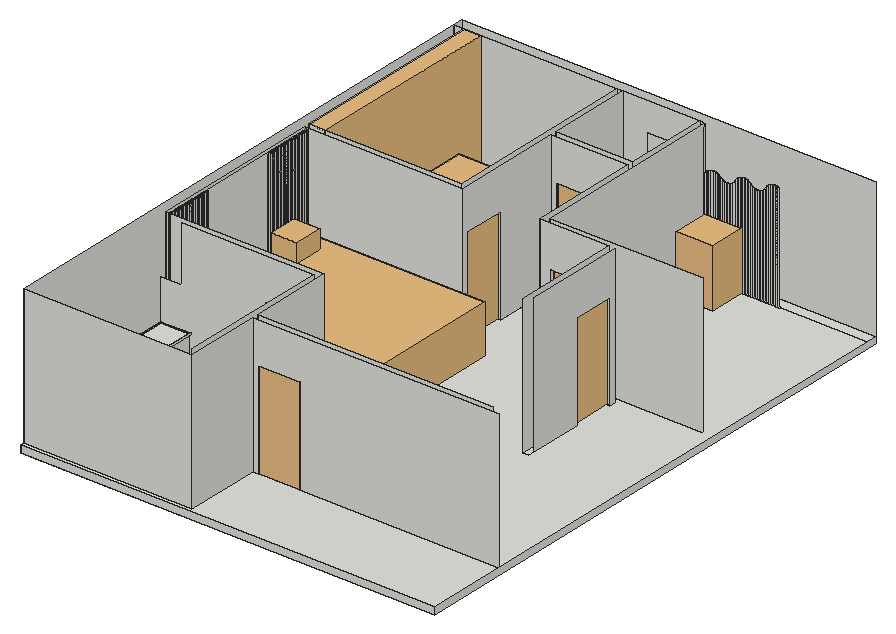
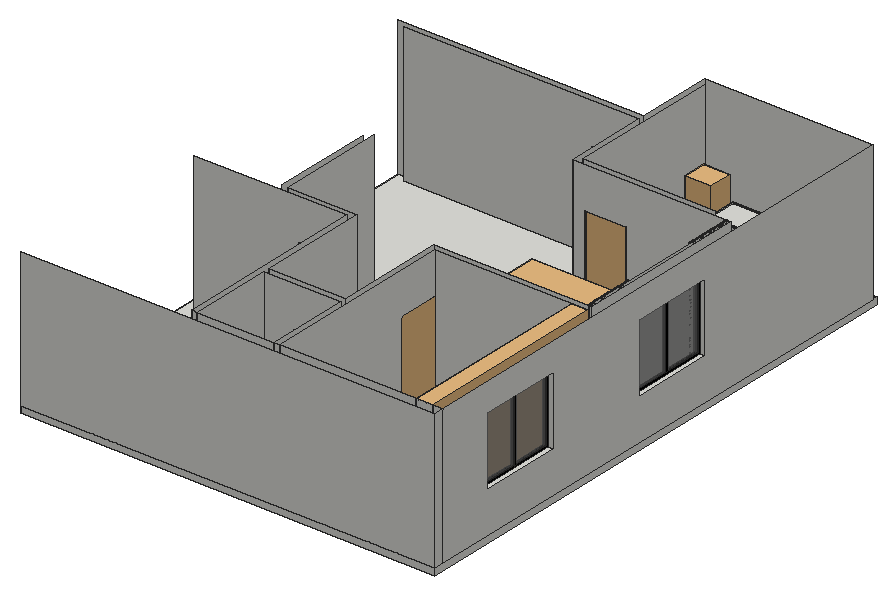
# SketchUp Ruby script. Lengths in inches.
U = 1.inch
M = Sketchup.active_model
def pt(a) = Geom::Point3d.new(a.map { |v| v * U })
def face(e, loops, mat)
  f = e.add_face(loops[0].map { |a| pt(a) })
  loops[1..].each { |l| e.add_face(l.map { |a| pt(a) }).erase! }
  f.material = f.back_material = mat if mat
  f
end
# faces: each face lists its corners as indices into pts; further lists are holes
def faces(e, pts, list, mat = nil) = list.each { |f| face(e, (f[0].is_a?(Array) ? f : [f]).map { |l| l.map { |i| pts[i] } }, mat) }
# xy, xz, yz: faces in a plane at the given z, y or x. An outline is a flat list of corners, or four numbers for a rectangle; further outlines are holes
def ring(l) = l.size == 4 ? [[l[0], l[1]], [l[2], l[1]], [l[2], l[3]], [l[0], l[3]]] : l.each_slice(2).to_a
def flat(e, list, mat, &to3) = list.each { |f| face(e, (f[0].is_a?(Array) ? f : [f]).map { |l| ring(l).map { |u, v| to3.(u, v) } }, mat) }
def xy(e, z, list, mat = nil) = flat(e, list, mat) { |x, y| [x, y, z] }
def xz(e, y, list, mat = nil) = flat(e, list, mat) { |x, z| [x, y, z] }
def yz(e, x, list, mat = nil) = flat(e, list, mat) { |y, z| [x, y, z] }
def lines(e, pts, list) = list.each { |a, b| e.add_line(pt(pts[a]), pt(pts[b])) }
# prism: a flat outline (further loops are holes) pulled along v
def prism(e, loops, v, mat = nil)
  f = face(e, loops, mat); d = Geom::Vector3d.new(v.map { |x| x * U })
  f.pushpull(f.normal.samedirection?(d) ? d.length : -d.length)
end
def box(e, o, s, mat = nil) = prism(e, [[o, [o[0] + s[0], o[1], o[2]], [o[0] + s[0], o[1] + s[1], o[2]], [o[0], o[1] + s[1], o[2]]]], [0, 0, s[2]], mat)
def at(x, y, z, deg = 0) = Geom::Transformation.translation(pt([x, y, z])) * Geom::Transformation.rotation(ORIGIN, Z_AXIS, deg.degrees)
def axes(o, x, y, z) = Geom::Transformation.new([*x, 0, *y, 0, *z, 0, *pt(o).to_a, 1])
def part(name) = M.definitions.add(name)
# library, detail: a bought-in or finely detailed component or shape, given as its bounding box
def library(name, o, s) = part(name).tap { |d| box(d.entities, o, s) }
def detail(e, o, s) = box(e.add_group.entities, o, s)
def put(e, d, t, mat = nil) = e.add_instance(d, t).tap { |i| i.material = mat if mat }
def group(e, t, mat = nil) = e.add_group.tap { |g| g.transformation = t; g.material = mat if mat }.entities
root = M.entities
M.materials.add("[Color_008]").color = [30, 30, 30]
M.materials.add("[Color_009]").color = [0, 0, 0]
M.materials.add("[Translucent_Glass_Gray]").color = [128, 128, 128]
M.materials["[Translucent_Glass_Gray]"].alpha = 0.5
c1 = part("Group\#1")
xy(c1.entities,0,[[0,0,82.68,1.18]],"[Color_009]")
xy(c1.entities,1.97,[[1.97,0.98,40.35,1.18],[42.32,0.98,80.71,1.18]])
xy(c1.entities,1.97,[[1.97,0,40.35,0.3],[42.32,0,80.71,0.3]],"[Color_009]")
xy(c1.entities,80.71,[[1.97,0,40.35,0.3],[42.32,0,80.71,0.3],[1.97,0.3,40.35,0.98],[42.32,0.3,80.71,0.98],[1.97,0.98,40.35,1.18],
  [42.32,0.98,80.71,1.18]])
xy(c1.entities,82.68,[[0,0,82.68,1.18]],"[Color_008]")
xz(c1.entities,0,[[[0,0,82.68,82.68],[1.97,1.97,40.35,80.71],[42.32,1.97,80.71,80.71]]],"[Color_009]")
xz(c1.entities,0.3,[[1.97,1.97,40.35,80.71],[42.32,1.97,80.71,80.71]],"[Translucent_Glass_Gray]")
xz(c1.entities,0.98,[[1.97,1.97,40.35,80.71],[42.32,1.97,80.71,80.71]],"[Translucent_Glass_Gray]")
xz(c1.entities,1.18,[[[0,0,82.68,82.68],[1.97,1.97,80.71,80.71]],[40.35,1.97,42.32,80.71]],"[Color_009]")
yz(c1.entities,0,[[0,0,1.18,82.68]],"[Color_009]")
yz(c1.entities,1.97,[[0.98,1.97,1.18,80.71]])
yz(c1.entities,1.97,[[0,1.97,0.3,80.71]],"[Color_009]")
yz(c1.entities,40.35,[[0,1.97,0.3,80.71],[0.98,1.97,1.18,80.71]],"[Color_009]")
yz(c1.entities,42.32,[[0,1.97,0.3,80.71],[0.98,1.97,1.18,80.71]])
yz(c1.entities,80.71,[[0,1.97,0.3,80.71],[0.98,1.97,1.18,80.71]],"[Color_009]")
yz(c1.entities,82.68,[[0,0,1.18,82.68]],"[Color_009]")
c2 = library("Curtain set",[2.63,-1.5,0.02],[153.32,14.06,114.15])
c3 = part("Vertical slat \#1")
box(c3.entities,[0,0,-18],[1,1,114])
c4 = part("Vertical slat")
box(c4.entities,[0,0,0],[1,1,96])
c5 = library("SKT_Nearly Natural 5' Kentia Palm Silk Tree",[-23.18,-17.61,0],[47.48,43.95,59.125])
c6 = library("Platform bed",[0,0,0],[83.59,112.46,35.43])
c7 = library("sofa+(2)",[-100.93,-81.02,-0.06],[174.43,145.32,46.54])
c8 = library("main+door",[0,-0.79,0],[47.24,7.88,82.68])
c9 = library("Component\#33",[0,0,0],[60.64,55.48,158.625])
c10 = library("CS300DRT",[0,0,0],[27.18,17.85,30.31])
xy(root,0,[[438.897,69.5,443.897,74.5],[428.897,141.5,433.897,146.5],[565.897,204,570.897,256.5],[565.897,292.5,570.897,297.5],[428.897,297.5,433.897,302.5],
  [433.897,297.5,438.897,302.5],[505.897,297.5,505.897,393.5,479.897,393.5,479.897,398.5,505.897,398.5,505.897,471,510.897,471,510.897,297.5],[510.897,297.5,515.897,302.5],[433.897,338.5,438.897,471],[438.897,393.5,443.897,398.5],
  [510.897,470,511.897,471],[512.097,470,513.097,471],[513.297,470,514.297,471],[514.497,470,515.497,471],[515.697,470,516.697,471],
  [516.897,470,517.897,471],[518.097,470,519.097,471],[519.297,470,520.297,471],[520.497,470,521.497,471],[521.697,470,522.697,471],
  [522.897,470,523.897,471],[524.097,470,525.097,471],[525.297,470,526.297,471],[526.497,470,527.497,471],[527.697,470,528.697,471],
  [528.897,470,529.897,471],[530.097,470,531.097,471],[531.297,470,532.297,471],[532.497,470,533.497,471],[533.697,470,534.697,471],
  [534.897,470,535.897,471],[536.097,470,537.097,471],[537.297,470,538.297,471],[538.497,470,539.497,471],[539.697,470,540.697,471],
  [540.897,470,541.897,471],[542.097,470,543.097,471],[543.297,470,544.297,471],[544.497,470,545.497,471],[545.697,470,546.697,471],
  [546.897,470,547.897,471],[548.097,470,549.097,471],[549.297,470,550.297,471],[550.497,470,551.497,471],[551.697,470,552.697,471],
  [552.897,470,553.897,471],[554.097,470,555.097,471],[555.297,470,556.297,471],[556.497,470,557.497,471],[557.697,470,558.697,471],
  [558.897,470,559.897,471],[560.097,470,561.097,471],[561.297,470,562.297,471],[562.497,470,563.497,471],[563.697,470,564.697,471],
  [564.897,470,565.897,471],[566.097,470,567.097,471],[567.297,470,568.297,471],[568.497,470,569.497,471],[569.697,470,570.697,471],
  [570.897,470,571.897,471],[572.097,470,573.097,471],[573.297,470,574.297,471],[574.497,470,575.497,471],[575.697,470,576.697,471],
  [292.397,471,652.397,480]])
xy(root,0.2,[[325.397,33.2,325.577,59.925],[325.397,60.325,325.577,87.05],[325.397,87.45,325.577,114.175],[325.397,114.575,325.577,141.3]])
xy(root,35.8,[[325.397,33.2,325.577,59.925],[325.397,60.325,325.577,87.05],[325.397,87.45,325.577,114.175],[325.397,114.575,325.577,141.3]])
xy(root,36,[[301.397,9,409.897,9,409.897,33,325.397,33,325.397,141.5,301.397,141.5],[325.397,33,327.397,141.5],[327.397,33,349.397,35],[349.397,33,385.897,35],[385.897,33,409.897,35],
  [292.397,186,301.397,258],[292.397,350.75,301.397,422.75]])
xz(root,3.625,[[292.397,0,438.897,120]])
xz(root,9,[[301.397,0,325.397,36],[325.397,0,409.897,36],[301.397,36,325.397,37],[325.397,36,409.897,37]])
xz(root,33,[[325.397,0,349.397,36],[349.397,0,385.897,12],[385.897,0,409.897,36],[349.397,12,385.897,24],[349.397,24,385.897,36]])
xz(root,33.2,[[325.397,0.2,325.577,35.8]])
xz(root,35,[[327.397,36,409.897,37]])
xz(root,59.925,[[325.397,0.2,325.577,35.8]])
xz(root,60.325,[[325.397,0.2,325.577,35.8]])
xz(root,69.5,[[438.897,0,443.897,0,443.897,84,479.897,84,479.897,0,652.397,0,652.397,120,438.897,120]])
xz(root,74.5,[[438.897,0,438.897,120,643.397,120,643.397,0,479.897,0,479.897,84,443.897,84,443.897,0]])
xz(root,87.05,[[325.397,0.2,325.577,35.8]])
xz(root,87.45,[[325.397,0.2,325.577,35.8]])
xz(root,114.175,[[325.397,0.2,325.577,35.8]])
xz(root,114.575,[[325.397,0.2,325.577,35.8]])
xz(root,141.3,[[325.397,0.2,325.577,35.8]])
xz(root,141.5,[[301.397,0,325.397,36],[325.397,0,392.897,0,392.897,84,428.897,84,428.897,0,433.897,0,433.897,120,319.217,120,319.217,72,301.397,72,301.397,37,327.397,37,327.397,36,325.397,36],[301.397,36,327.397,37]])
xz(root,146.5,[[301.397,0,301.397,120,438.897,120,438.897,0,428.897,0,428.897,84,392.897,84,392.897,0]])
xz(root,186,[[292.397,36,301.397,96]])
xz(root,256.5,[[565.897,0,570.897,84]])
xz(root,258,[[292.397,36,301.397,96]])
xz(root,292.5,[[565.897,0,570.897,84]])
xz(root,297.5,[[301.397,0,438.897,120],[505.897,0,515.897,0,515.897,84,551.897,84,551.897,0,565.897,0,565.897,120,505.897,120]])
xz(root,302.5,[[301.397,0,433.897,120],[433.897,0,438.897,84],[510.897,0,510.897,120,643.397,120,643.397,0,551.897,0,551.897,84,515.897,84,515.897,0]])
xz(root,338.5,[[433.897,0,438.897,84]])
xz(root,350.75,[[292.397,36,301.397,96]])
xz(root,393.5,[[438.897,0,443.897,0,443.897,84,479.897,84,479.897,0,505.897,0,505.897,120,438.897,120]])
xz(root,398.5,[[438.897,0,438.897,120,505.897,120,505.897,0,479.897,0,479.897,84,443.897,84,443.897,0]])
xz(root,422.75,[[292.397,36,301.397,96]])
xz(root,470,[[510.897,0,511.897,0,511.897,82.696,511.848,82.623,511.778,82.516,511.709,82.408,511.642,82.299,511.577,82.189,511.514,82.078,511.453,81.965,511.393,81.852,511.335,81.738,511.279,81.623,511.225,81.507,511.172,81.39,511.122,81.273,511.073,81.154,511.026,81.035,510.981,80.915,510.938,80.795,510.897,80.674],[512.097,0,513.097,0,513.097,84.081,513.094,84.078,513,83.991,512.908,83.902,512.728,83.72,512.64,83.627,512.554,83.532,512.469,83.436,512.386,83.339,512.304,83.241,512.224,83.141,512.146,83.04,512.097,82.976],[513.297,0,514.297,0,514.297,84.991,514.209,84.935,514.101,84.865,513.995,84.794,513.89,84.721,513.786,84.646,513.683,84.57,513.582,84.492,513.482,84.412,513.383,84.331,513.297,84.258],[514.497,0,515.497,0,515.497,85.601,515.456,85.584,515.338,85.535,515.221,85.483,515.105,85.429,514.989,85.374,514.875,85.316,514.761,85.257,514.649,85.196,514.537,85.134,514.497,85.11],[515.697,0,516.697,0,516.697,85.984,516.672,85.978,516.548,85.948,516.424,85.915,516.301,85.881,516.178,85.844,516.056,85.806,515.935,85.765,515.814,85.723,515.697,85.68],
  [516.897,0,517.897,0,517.897,86.171,517.808,86.164,517.681,86.151,517.554,86.136,517.427,86.12,517.3,86.101,517.174,86.081,517.048,86.058,516.922,86.033,516.897,86.028],[518.097,0,519.097,0,519.097,86.176,519.086,86.177,518.959,86.185,518.831,86.191,518.703,86.194,518.575,86.196,518.447,86.196,518.319,86.193,518.191,86.189,518.097,86.184],[519.297,0,520.297,0,520.297,85.999,520.226,86.015,520.101,86.041,519.975,86.065,519.849,86.087,519.722,86.107,519.596,86.125,519.469,86.141,519.342,86.155,519.297,86.159],[520.497,0,521.497,0,521.497,85.629,521.45,85.647,521.331,85.693,521.21,85.736,521.089,85.778,520.968,85.818,520.846,85.856,520.723,85.892,520.599,85.926,520.497,85.952],[521.697,0,522.697,0,522.697,85.032,522.601,85.09,522.49,85.154,522.378,85.216,522.265,85.276,522.151,85.335,522.037,85.391,521.921,85.446,521.805,85.499,521.697,85.546],
  [522.897,0,523.897,0,523.897,83.953,523.873,83.981,523.785,84.085,523.698,84.191,523.613,84.298,523.53,84.407,523.448,84.516,523.347,84.594,523.244,84.67,523.139,84.744,523.034,84.817,522.927,84.887,522.897,84.906],[524.097,0,525.097,0,525.097,82.807,525.051,82.844,524.945,82.93,524.84,83.018,524.736,83.107,524.635,83.198,524.534,83.291,524.435,83.385,524.337,83.48,524.241,83.578,524.147,83.676,524.097,83.729],[525.297,0,526.297,0,526.297,82.013,526.181,82.078,526.0625,82.146,525.945,82.217,525.829,82.289,525.714,82.363,525.601,82.439,525.488,82.516,525.377,82.596,525.297,82.654],[526.497,0,527.497,0,527.497,81.467,527.416,81.497,527.289,81.547,527.162,81.598,527.036,81.651,526.911,81.706,526.787,81.763,526.664,81.823,526.541,81.884,526.497,81.906],[527.697,0,528.697,0,528.697,81.123,528.593,81.145,528.46,81.176,528.328,81.209,528.195,81.244,528.064,81.281,527.933,81.32,527.803,81.362,527.697,81.397],
  [528.897,0,529.897,0,529.897,80.955,529.808,80.962,529.672,80.974,529.536,80.988,529.4,81.004,529.265,81.022,529.13,81.042,528.995,81.065,528.897,81.083],[530.097,0,531.097,0,531.097,80.955,531.037,80.95,530.9,80.943,530.764,80.938,530.627,80.935,530.491,80.934,530.354,80.935,530.217,80.939,530.097,80.944],[531.297,0,532.297,0,532.297,81.121,532.255,81.112,532.121,81.085,531.987,81.061,531.852,81.039,531.717,81.019,531.581,81.001,531.445,80.985,531.309,80.971,531.297,80.97],[532.497,0,533.497,0,533.497,81.464,533.439,81.442,533.31,81.397,533.18,81.354,533.049,81.314,532.918,81.275,532.787,81.238,532.655,81.203,532.522,81.171,532.497,81.165],[533.697,0,534.697,0,534.697,82.007,534.684,82,534.564,81.936,534.442,81.873,534.32,81.8125,534.197,81.754,534.072,81.697,533.947,81.642,533.821,81.589,533.697,81.539],
  [534.897,0,535.897,0,535.897,82.8,535.828,82.745,535.719,82.663,535.609,82.582,535.497,82.503,535.385,82.426,535.271,82.35,535.156,82.277,535.04,82.205,534.922,82.135,534.897,82.12],[536.097,0,537.097,0,537.097,83.942,537.027,83.861,536.935,83.759,536.842,83.66,536.747,83.561,536.651,83.464,536.553,83.369,536.454,83.275,536.353,83.183,536.251,83.092,536.147,83.003,536.097,82.961],[537.297,0,538.297,0,538.297,86.14,538.287,86.123,538.222,86.013,538.159,85.902,538.097,85.79,538.038,85.676,537.98,85.5625,537.924,85.447,537.869,85.331,537.817,85.215,537.767,85.097,537.718,84.979,537.671,84.859,537.626,84.74,537.583,84.619,537.542,84.498,537.461,84.388,537.377,84.28,537.297,84.18],[538.497,0,539.497,0,539.497,87.671,539.462,87.636,539.373,87.544,539.285,87.451,539.199,87.356,539.114,87.261,539.031,87.163,538.949,87.065,538.869,86.965,538.791,86.864,538.714,86.762,538.638,86.658,538.565,86.553,538.497,86.454],[539.697,0,540.697,0,540.697,88.657,540.64,88.618,540.535,88.545,540.431,88.47,540.328,88.394,540.227,88.316,540.127,88.236,540.028,88.155,539.93,88.072,539.834,87.988,539.739,87.902,539.697,87.863],
  [540.897,0,541.897,0,541.897,89.321,541.866,89.307,541.75,89.253,541.634,89.198,541.52,89.141,541.406,89.081,541.294,89.021,541.182,88.958,541.072,88.893,540.962,88.827,540.897,88.787],[542.097,0,543.097,0,543.097,89.747,543.069,89.739,542.946,89.705,542.823,89.668,542.701,89.63,542.58,89.589,542.459,89.547,542.339,89.503,542.219,89.457,542.101,89.409,542.097,89.407],[543.297,0,544.297,0,544.297,89.972,544.198,89.961,544.071,89.944,543.945,89.926,543.819,89.905,543.693,89.882,543.567,89.858,543.442,89.831,543.317,89.802,543.297,89.798],[544.497,0,545.497,0,545.497,90.014,545.476,90.015,545.348,90.019,545.22,90.02,545.092,90.02,544.964,90.018,544.836,90.013,544.708,90.007,544.58,89.998,544.497,89.992],[545.697,0,546.697,0,546.697,89.875,546.62,89.89,546.494,89.912,546.367,89.932,546.241,89.95,546.114,89.966,545.986,89.979,545.859,89.991,545.731,90.001,545.697,90.003],
  [546.897,0,547.897,0,547.897,89.545,547.855,89.561,547.734,89.602,547.613,89.642,547.49,89.68,547.368,89.716,547.244,89.75,547.12,89.782,546.996,89.812,546.897,89.834],[548.097,0,549.097,0,549.097,88.999,549.023,89.04,548.91,89.1,548.796,89.159,548.682,89.216,548.566,89.271,548.45,89.324,548.332,89.375,548.214,89.424,548.097,89.471],[549.297,0,550.297,0,550.297,88.073,550.258,88.123,550.175,88.231,550.093,88.341,549.992,88.418,549.888,88.494,549.784,88.568,549.679,88.641,549.572,88.712,549.464,88.781,549.356,88.848,549.297,88.883],[550.497,0,551.497,0,551.497,86.831,551.485,86.842,551.381,86.931,551.279,87.022,551.179,87.115,551.08,87.209,550.982,87.305,550.886,87.402,550.792,87.501,550.699,87.601,550.607,87.702,550.518,87.805,550.497,87.829],[551.697,0,552.697,0,552.697,85.977,552.59,86.041,552.474,86.113,552.359,86.187,552.246,86.263,552.133,86.341,552.022,86.42,551.912,86.501,551.803,86.584,551.697,86.667],
  [552.897,0,553.897,0,553.897,85.385,553.807,85.422,553.681,85.475,553.556,85.531,553.432,85.588,553.309,85.647,553.186,85.708,553.065,85.771,552.897,85.862],[554.097,0,555.097,0,555.097,85.002,554.972,85.033,554.84,85.068,554.709,85.105,554.578,85.145,554.448,85.186,554.318,85.229,554.189,85.274,554.097,85.308],[555.297,0,556.297,0,556.297,84.8,556.181,84.812,556.045,84.828,555.91,84.846,555.775,84.867,555.64,84.889,555.506,84.914,555.372,84.941,555.297,84.957],[556.497,0,557.497,0,557.497,84.766,557.409,84.762,557.272,84.759,557.136,84.758,556.999,84.76,556.862,84.763,556.726,84.768,556.589,84.776,556.497,84.783],[557.697,0,558.697,0,558.697,84.897,558.631,84.885,558.497,84.863,558.361,84.843,558.226,84.825,558.09,84.809,557.954,84.796,557.818,84.784,557.697,84.776],
  [558.897,0,559.897,0,559.897,85.203,559.825,85.179,559.694,85.138,559.563,85.099,559.432,85.062,559.3,85.028,559.167,84.995,559.034,84.964,558.9,84.936,558.897,84.935],[560.097,0,561.097,0,561.097,85.703,561.087,85.697,560.965,85.637,560.842,85.578,560.717,85.521,560.592,85.466,560.466,85.413,560.339,85.362,560.212,85.313,560.097,85.272],[561.297,0,562.297,0,562.297,86.438,562.254,86.406,562.142,86.327,562.03,86.25,561.916,86.175,561.801,86.101,561.684,86.029,561.567,85.959,561.449,85.891,561.329,85.824,561.297,85.807],[562.497,0,563.497,0,563.497,87.495,563.487,87.484,563.392,87.385,563.296,87.288,563.198,87.193,563.099,87.099,562.998,87.007,562.896,86.916,562.792,86.827,562.687,86.74,562.581,86.654,562.497,86.589],[563.697,0,564.697,0,564.697,89.529,564.683,89.501,564.625,89.387,564.569,89.272,564.514,89.156,564.462,89.039,564.411,88.921,564.363,88.803,564.316,88.684,564.271,88.564,564.228,88.443,564.187,88.322,564.106,88.213,564.022,88.104,563.937,87.997,563.85,87.892,563.762,87.788,563.697,87.715],
  [564.897,0,565.897,0,565.897,91.239,565.844,91.181,565.759,91.085,565.676,90.988,565.594,90.889,565.514,90.789,565.435,90.688,565.359,90.586,565.283,90.482,565.21,90.378,565.138,90.272,565.067,90.165,564.999,90.057,564.932,89.948,564.897,89.889],[566.097,0,567.097,0,567.097,92.31,567.076,92.295,566.973,92.218,566.872,92.14,566.772,92.06,566.673,91.979,566.575,91.897,566.479,91.812,566.384,91.726,566.29,91.639,566.198,91.55,566.107,91.46,566.097,91.45],[567.297,0,568.297,0,568.297,93.031,568.165,92.965,568.051,92.906,567.939,92.845,567.827,92.782,567.716,92.718,567.607,92.651,567.499,92.583,567.391,92.514,567.297,92.451],[568.497,0,569.497,0,569.497,93.501,569.468,93.493,569.346,93.454,569.224,93.414,569.104,93.371,568.984,93.327,568.864,93.281,568.746,93.233,568.628,93.183,568.511,93.131,568.497,93.125],[569.697,0,570.697,0,570.697,93.766,570.59,93.75,570.463,93.729,570.337,93.707,570.212,93.682,570.087,93.655,569.962,93.627,569.838,93.596,569.714,93.564,569.697,93.559],
  [570.897,0,571.897,0,571.897,93.844,571.865,93.845,571.737,93.844,571.609,93.842,571.481,93.837,571.353,93.831,571.225,93.823,571.098,93.812,570.97,93.8,570.897,93.791],[572.097,0,573.097,0,573.097,93.742,573.012,93.756,572.886,93.774,572.759,93.79,572.631,93.804,572.504,93.816,572.376,93.825,572.249,93.833,572.121,93.839,572.097,93.84],[573.297,0,574.297,0,574.297,93.453,574.258,93.466,574.135,93.504,574.012,93.54,573.889,93.574,573.765,93.606,573.641,93.636,573.516,93.664,573.39,93.69,573.297,93.708],[574.497,0,575.497,0,575.497,92.954,575.441,92.983,575.327,93.04,575.211,93.095,575.094,93.148,574.977,93.199,574.859,93.248,574.74,93.296,574.621,93.341,574.5,93.385,574.497,93.386]])
xz(root,471,[[292.397,0,301.397,120],[301.397,0,433.897,120],[433.897,0,438.897,120],[[438.897,0,505.897,120],[460.397,72,484.397,96]],[505.897,0,510.897,120]])
xz(root,480,[[292.397,0,652.397,120]])
yz(root,292.397,[[[3.625,0,471,120],[350.75,36,422.75,96],[186,36,258,96]],[471,0,480,120]])
yz(root,301.397,[[9,0,141.5,36],[[146.5,0,297.5,120],[186,36,258,96]],[[302.5,0,471,120],[350.75,36,422.75,96]],[9,36,141.5,37]])
yz(root,325.397,[[[33,0,141.5,36],[114.575,0.2,141.3,35.8],[87.45,0.2,114.175,35.8],[33.2,0.2,59.925,35.8],[60.325,0.2,87.05,35.8]]])
yz(root,325.577,[[33.2,0.2,59.925,35.8],[60.325,0.2,87.05,35.8],[87.45,0.2,114.175,35.8],[114.575,0.2,141.3,35.8]])
yz(root,327.397,[[35,36,141.5,37]])
yz(root,392.897,[[141.5,0,146.5,84]])
yz(root,409.897,[[9,0,33,36],[9,36,35,37]])
yz(root,428.897,[[141.5,0,146.5,84]])
yz(root,433.897,[[9,0,141.5,120],[338.5,0,338.5,84,302.5,84,302.5,120,471,120,471,0]])
yz(root,438.897,[[3.625,0,69.5,120],[74.5,0,146.5,120],[297.5,0,302.5,0,302.5,84,338.5,84,338.5,0,393.5,0,393.5,120,297.5,120],[398.5,0,471,120]])
yz(root,443.897,[[69.5,0,74.5,84],[393.5,0,398.5,84]])
yz(root,479.897,[[69.5,0,74.5,84],[393.5,0,398.5,84]])
yz(root,505.897,[[297.5,0,393.5,120],[398.5,0,471,120]])
yz(root,510.897,[[302.5,0,470,120],[470,0,471,120]])
yz(root,515.897,[[297.5,0,302.5,84]])
yz(root,551.897,[[297.5,0,302.5,84]])
yz(root,565.897,[[204,0,204,120,297.5,120,297.5,0,292.5,0,292.5,84,256.5,84,256.5,0]])
yz(root,570.897,[[210,0,256.5,0,256.5,84,292.5,84,292.5,0,297.5,0,297.5,120,210,120]])
p = [[409.897,33,0],[433.897,33,0],[433.897,9,0],[409.897,9,0]]
lines(root,p,[[0,1],[2,3]])
put(root,c1,axes([299.91,350.75,36],[0,0.87086,0],[-2.552,0,0],[0,0,0.72571]))
put(root,c1,axes([299.91,186,36],[0,0.87086,0],[-2.552,0,0],[0,0,0.72571]))
put(root,c2,axes([313.95,299.61,5.83],[0,1.09899,0],[-1,0,0],[0,0,1]))
g1 = group(root,at(304.49,146.5,0))
xy(g1,6,[[0,12,18,139]])
xy(g1,24,[[0,12,18,139]])
xz(g1,12,[[0,6,18,24]])
xz(g1,139,[[0,6,18,24]])
yz(g1,0,[[0,0,151,5.91],[[0,5.91,151,120],[99.22,6,139,24]],[99.22,6,100.22,24],[100.22,6,139,24]])
yz(g1,18,[[[12,6,139,24],[13,7,138,23]],[[13,7,44.25,23],[13.2,7.2,44.05,22.8]],[[44.25,7,75.5,23],[44.45,7.2,75.3,22.8]],[[75.5,7,106.75,23],[75.7,7.2,106.55,22.8]],[[106.75,7,138,23],[106.95,7.2,137.8,22.8]],
  [13.2,7.2,44.05,22.8],[44.45,7.2,75.3,22.8],[75.7,7.2,106.55,22.8],[106.95,7.2,137.8,22.8]])
put(g1,c3,at(0,1.23,24))
put(g1,c3,at(0,145.23,24))
put(g1,c3,at(0,146.43,24))
put(g1,c3,at(0,147.63,24))
put(g1,c3,at(0,148.83,24))
put(g1,c3,at(0,140.43,24))
put(g1,c4,at(0,138.03,24))
put(g1,c4,at(0,112.83,24))
put(g1,c4,at(0,110.43,24))
put(g1,c4,at(0,109.23,24))
put(g1,c4,at(0,114.03,24))
put(g1,c4,at(0,108.03,24))
put(g1,c4,at(0,115.23,24))
put(g1,c4,at(0,116.43,24))
put(g1,c4,at(0,118.83,24))
put(g1,c4,at(0,117.63,24))
put(g1,c4,at(0,120.03,24))
put(g1,c4,at(0,121.23,24))
put(g1,c4,at(0,122.43,24))
put(g1,c4,at(0,111.63,24))
put(g1,c4,at(0,106.83,24))
put(g1,c3,at(0,139.23,24))
put(g1,c3,at(0,142.83,24))
put(g1,c3,at(0,8.43,24))
put(g1,c4,at(0,19.23,24))
put(g1,c4,at(0,22.83,24))
put(g1,c4,at(0,27.63,24))
put(g1,c4,at(0,26.43,24))
put(g1,c4,at(0,14.43,24))
put(g1,c3,at(0,10.83,24))
put(g1,c4,at(0,15.63,24))
put(g1,c4,at(0,28.83,24))
put(g1,c4,at(0,36.03,24))
put(g1,c3,at(0,2.43,24))
put(g1,c4,at(0,32.43,24))
put(g1,c4,at(0,21.63,24))
put(g1,c3,at(0,144.03,24))
put(g1,c4,at(0,25.23,24))
put(g1,c4,at(0,33.63,24))
put(g1,c4,at(0,12.03,24))
put(g1,c4,at(0,31.23,24))
put(g1,c3,at(0,6.03,24))
put(g1,c4,at(0,13.23,24))
put(g1,c4,at(0,24.03,24))
put(g1,c4,at(0,37.23,24))
put(g1,c4,at(0,38.43,24))
put(g1,c3,at(0,7.23,24))
put(g1,c4,at(0,16.83,24))
put(g1,c4,at(0,18.03,24))
put(g1,c4,at(0,20.43,24))
put(g1,c4,at(0,30.03,24))
put(g1,c3,at(0,9.63,24))
put(g1,c4,at(0,39.63,24))
put(g1,c4,at(0,34.83,24))
put(g1,c3,at(0,4.83,24))
put(g1,c3,at(0,3.63,24))
put(g1,c4,at(0,132.03,24))
put(g1,c4,at(0,136.83,24))
put(g1,c4,at(0,129.63,24))
put(g1,c4,at(0,130.83,24))
put(g1,c4,at(0,127.23,24))
put(g1,c4,at(0,128.43,24))
put(g1,c4,at(0,133.23,24))
put(g1,c4,at(0,134.43,24))
put(g1,c4,at(0,135.63,24))
put(g1,c4,at(0,126.03,24))
put(g1,c3,at(0,141.63,24))
put(g1,c4,at(0,123.63,24))
put(g1,c4,at(0,124.83,24))
g2 = group(g1,at(0,0.03,24))
box(g2,[0,0,-18.09],[1,1,114.09])
put(root,c5,axes([314.49,265.68,24],[0.5695,0,0],[0,0.5695,0],[0,0,0.5695]))
put(root,c5,axes([319.76,19.16,36.45],[0.5,0,0],[0,0.5,0],[0,0,0.5]))
put(root,c6,axes([406.04,447.1,0],[-1.08,0,0],[0,-1.08,0],[0,0,1.08]))
put(root,c7,axes([395.52,235.12,0.05],[0.9,0,0],[0,0.9,0],[0,0,0.9]))
put(root,c8,axes([392.9,142.32,0],[0.762,0,0],[0,0.31,0],[0,0,1.016]))
put(root,c9,axes([432.71,33,0],[-0.3762,0,0],[0,-0.3762,0],[0,0,0.3762]))
put(root,c8,axes([436.09,302.82,0],[0,0.762,0],[-0.31,0,0],[0,0,1.016]))
put(root,c10,axes([438.9,428.27,0],[1.26,0,0],[0,1.26,0],[0,0,1.26]))
put(root,c8,axes([443.9,394.32,0],[0.762,0,0],[0,0.31,0],[0,0,1.016]))
put(root,c8,axes([443.9,70.32,0],[0.762,0,0],[0,0.31,0],[0,0,1.016]))
g3 = group(root,at(292.4,0,-6))
box(g3,[0,0,0],[360,480,6])
put(root,c5,axes([522.98,453.35,0],[0.85,0,0],[0,0.85,0],[0,0,0.85]))
put(root,c8,axes([515.9,300.91,0],[0.762,0,0],[0,0.31,0],[0,0,1.016]))
put(root,c8,axes([568.09,256.5,0],[0,0.762,0],[-0.31,0,0],[0,0,1.016]))
